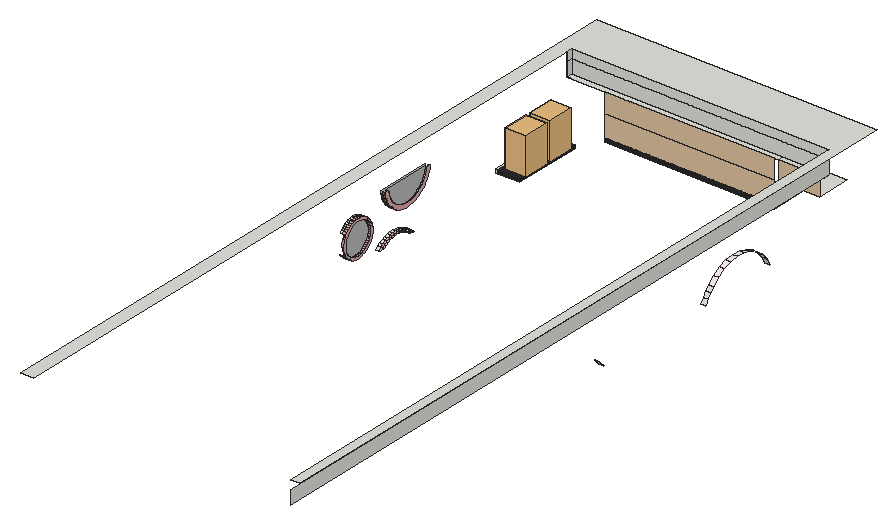
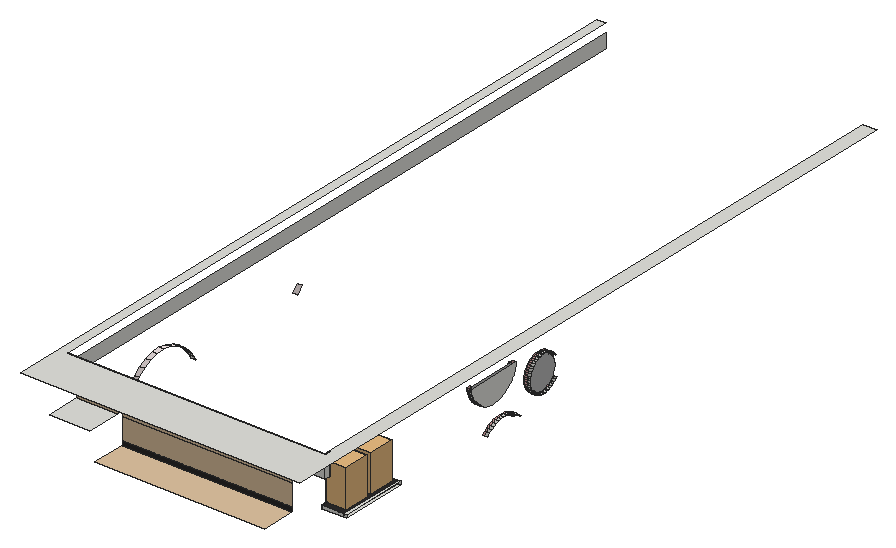
# SketchUp Ruby script. Lengths in inches.
U = 1.inch
M = Sketchup.active_model
def pt(a) = Geom::Point3d.new(a.map { |v| v * U })
def face(e, loops, mat)
  f = e.add_face(loops[0].map { |a| pt(a) })
  loops[1..].each { |l| e.add_face(l.map { |a| pt(a) }).erase! }
  f.material = f.back_material = mat if mat
  f
end
# faces: each face lists its corners as indices into pts; further lists are holes
def faces(e, pts, list, mat = nil) = list.each { |f| face(e, (f[0].is_a?(Array) ? f : [f]).map { |l| l.map { |i| pts[i] } }, mat) }
# xy, xz, yz: faces in a plane at the given z, y or x. An outline is a flat list of corners, or four numbers for a rectangle; further outlines are holes
def ring(l) = l.size == 4 ? [[l[0], l[1]], [l[2], l[1]], [l[2], l[3]], [l[0], l[3]]] : l.each_slice(2).to_a
def flat(e, list, mat, &to3) = list.each { |f| face(e, (f[0].is_a?(Array) ? f : [f]).map { |l| ring(l).map { |u, v| to3.(u, v) } }, mat) }
def xy(e, z, list, mat = nil) = flat(e, list, mat) { |x, y| [x, y, z] }
def xz(e, y, list, mat = nil) = flat(e, list, mat) { |x, z| [x, y, z] }
def yz(e, x, list, mat = nil) = flat(e, list, mat) { |y, z| [x, y, z] }
def lines(e, pts, list) = list.each { |a, b| e.add_line(pt(pts[a]), pt(pts[b])) }
# prism: a flat outline (further loops are holes) pulled along v
def prism(e, loops, v, mat = nil)
  f = face(e, loops, mat); d = Geom::Vector3d.new(v.map { |x| x * U })
  f.pushpull(f.normal.samedirection?(d) ? d.length : -d.length)
end
def box(e, o, s, mat = nil) = prism(e, [[o, [o[0] + s[0], o[1], o[2]], [o[0] + s[0], o[1] + s[1], o[2]], [o[0], o[1] + s[1], o[2]]]], [0, 0, s[2]], mat)
def at(x, y, z, deg = 0) = Geom::Transformation.translation(pt([x, y, z])) * Geom::Transformation.rotation(ORIGIN, Z_AXIS, deg.degrees)
def axes(o, x, y, z) = Geom::Transformation.new([*x, 0, *y, 0, *z, 0, *pt(o).to_a, 1])
def part(name) = M.definitions.add(name)
# library, detail: a bought-in or finely detailed component or shape, given as its bounding box
def library(name, o, s) = part(name).tap { |d| box(d.entities, o, s) }
def detail(e, o, s) = box(e.add_group.entities, o, s)
def put(e, d, t, mat = nil) = e.add_instance(d, t).tap { |i| i.material = mat if mat }
def group(e, t, mat = nil) = e.add_group.tap { |g| g.transformation = t; g.material = mat if mat }.entities
root = M.entities
M.materials.add("Generic").color = [224, 169, 169]
M.materials.add("Generic\#1").color = [44, 42, 42]
M.materials.add("Generic\#2").color = [246, 234, 234]
M.materials.add("Generic\#3").color = [224, 196, 161]
M.materials.add("[Mirror 01]").color = [185, 185, 185]
c1 = library("Untitled (9)",[-0.59,0,0],[15.67,17.07,16.5])
xy(root,88.25,[[9,393.02,10.6875,439.14]])
xy(root,88.25,[[10.6875,393.02,25.625,439.14]],"Generic\#1")
xy(root,89.18,[[34.875,453.375,150.375,476.6875]],"Generic\#3")
xy(root,90.4375,[[9,393.02,10.6875,439.14]])
xy(root,90.4375,[[10.6875,393.02,25.625,439.14]],"Generic\#1")
xy(root,107.14,[[153.2,453.375,180.77,476.9375]])
xy(root,120,[[10.6875,453.375,153.2,453.375,153.2,457.3,9,457.3,9,453.625,10.6875,453.625],[9,453.375,10.6875,453.625],[153.2,453.375,184.0625,457.3]])
xy(root,135.25,[[184.0625,0,190,0,190,490.125,0,490.125,0,0.4375,9,0.4375,9,457.3,184.0625,457.3]])
xz(root,393.02,[[9,88.25,10.6875,90.4375]])
xz(root,393.02,[[10.6875,88.25,25.625,90.4375]],"Generic\#1")
xz(root,439.14,[[9,88.25,10.6875,90.4375],[10.6875,88.25,25.625,90.4375]])
xz(root,453.375,[[34.875,89.18,149.93,92.07]],"Generic\#1")
xz(root,453.375,[[34.875,92.07,149.93,106.62],[34.875,106.62,149.93,120],[153.2,107.14,180.77,120]],"Generic\#3")
xz(root,457.3,[[9,120,184.0625,129.25],[9,129.25,184.0625,135.25]])
yz(root,9,[[314.19,103.09,315.21,103.12,316.22,103.2,317.23,103.34,318.23,103.52,319.22,103.77,320.19,104.06,321.15,104.41,322.09,104.8,323,105.25,323.89,105.74,324.75,106.28,325.59,106.87,326.39,107.5,327.15,108.17,327.88,108.875,328.57,109.625,329.22,110.41,329.82,111.23,330.38,112.07,330.9,112.95,331.37,113.85,331.79,114.78,332.15,115.73,332.47,116.7,332.74,117.68,332.95,118.67,333.16,120,295.22,120,295.4375,118.67,295.65,117.68,295.91,116.7,296.23,115.73,296.6,114.78,297.02,113.85,297.49,112.95,298,112.07,298.56,111.23,299.17,110.41,299.82,109.625,300.51,108.875,301.24,108.17,302,107.5,302.8,106.87,303.63,106.28,304.49,105.74,305.38,105.25,306.3,104.8,307.24,104.41,308.19,104.06,309.17,103.77,310.15,103.52,311.15,103.34,312.16,103.2,313.18,103.12],[453.375,120,453.625,129.25],[453.625,120,457.3,129.25],[453.375,129.25,453.625,135.25],[453.625,129.25,457.3,135.25]])
yz(root,10.6875,[[271.54,91.83,272.78,91.92,274,92.15,275.18,92.52,276.32,93.03,277.39,93.66,278.38,94.4,279.28,95.26,280.08,96.21,280.76,97.25,281.32,98.36,281.75,99.52,282.04,100.73,282.2,101.96,282.21,103.2,282.08,104.4375,281.8125,105.65,281.41,106.82,280.875,107.94,280.21,109,279.4375,109.97,278.56,110.84,277.58,111.61,276.53,112.26,275.4,112.79,274.23,113.1875,273.01,113.45,271.78,113.57,270.53,113.54,269.3,113.38,268.1,113.08,266.9375,112.64,265.83,112.07,264.8,111.38,263.85,110.58,263,109.67,262.26,108.68,261.64,107.6,261.14,106.47,260.78,105.28,260.56,104.06,260.47,102.82,260.53,101.58,260.73,100.35,261.07,99.16,261.54,98.01,262.14,96.92,262.85,95.91,263.68,94.98,264.61,94.16,265.63,93.45,266.72,92.86,267.875,92.39,269.07,92.07,270.3,91.875],[314.19,105.5625,315.08,105.59,315.96,105.66,316.84,105.77,317.71,105.9375,318.57,106.15,319.42,106.41,320.25,106.71,321.07,107.05,321.86,107.4375,322.64,107.87,323.39,108.34,324.11,108.85,324.81,109.4,325.47,109.98,326.11,110.6,326.71,111.25,327.27,111.93,327.8,112.64,328.29,113.38,328.74,114.14,329.14,114.93,329.51,115.74,329.83,116.5625,330.11,117.4,330.34,118.26,330.52,119.125,330.66,120,297.72,120,297.86,119.125,298.05,118.26,298.28,117.4,298.56,116.5625,298.88,115.74,299.24,114.93,299.65,114.14,300.1,113.38,300.59,112.64,301.12,111.93,301.68,111.25,302.28,110.6,302.91,109.98,303.58,109.4,304.28,108.85,305,108.34,305.75,107.87,306.52,107.4375,307.32,107.05,308.14,106.71,308.97,106.41,309.82,106.15,310.68,105.9375,311.55,105.77,312.43,105.66,313.31,105.59]],"[Mirror 01]")
yz(root,12.1875,[[314.19,103.09,315.21,103.12,316.22,103.2,317.23,103.34,318.23,103.52,319.22,103.77,320.19,104.06,321.15,104.41,322.09,104.8,323,105.25,323.89,105.74,324.75,106.28,325.59,106.87,326.39,107.5,327.15,108.17,327.88,108.875,328.57,109.625,329.22,110.41,329.82,111.23,330.38,112.07,330.9,112.95,331.37,113.85,331.79,114.78,332.15,115.73,332.47,116.7,332.74,117.68,332.95,118.67,333.16,120,330.66,120,330.52,119.125,330.34,118.26,330.11,117.4,329.83,116.5625,329.51,115.74,329.14,114.93,328.74,114.14,328.29,113.38,327.8,112.64,327.27,111.93,326.71,111.25,326.11,110.6,325.47,109.98,324.81,109.4,324.11,108.85,323.39,108.34,322.64,107.87,321.86,107.4375,321.07,107.05,320.25,106.71,319.42,106.41,318.57,106.15,317.71,105.9375,316.84,105.77,315.96,105.66,315.08,105.59,314.19,105.5625,313.31,105.59,312.43,105.66,311.55,105.77,310.68,105.9375,309.82,106.15,308.97,106.41,308.14,106.71,307.32,107.05,306.52,107.4375,305.75,107.87,305,108.34,304.28,108.85,303.58,109.4,302.91,109.98,302.28,110.6,301.68,111.25,301.12,111.93,300.59,112.64,300.1,113.38,299.65,114.14,299.24,114.93,298.88,115.74,298.56,116.5625,298.28,117.4,298.05,118.26,297.86,119.125,297.72,120,295.22,120,295.4375,118.67,295.65,117.68,295.91,116.7,296.23,115.73,296.6,114.78,297.02,113.85,297.49,112.95,298,112.07,298.56,111.23,299.17,110.41,299.82,109.625,300.51,108.875,301.24,108.17,302,107.5,302.8,106.87,303.63,106.28,304.49,105.74,305.38,105.25,306.3,104.8,307.24,104.41,308.19,104.06,309.17,103.77,310.15,103.52,311.15,103.34,312.16,103.2,313.18,103.12]],"Generic")
yz(root,12.9375,[[[271.5625,90.52,272.95,90.625,274.32,90.89,275.64,91.3,276.91,91.86,278.11,92.57,279.22,93.41,280.23,94.37,281.125,95.43,281.89,96.59,282.52,97.84,283,99.14,283.33,100.49,283.5,101.87,283.52,103.26,283.37,104.65,283.07,106,282.62,107.32,282.02,108.57,281.28,109.75,280.41,110.84,279.42,111.82,278.33,112.68,277.15,113.41,275.89,114,274.57,114.45,273.21,114.74,271.83,114.87,270.4375,114.85,269.06,114.66,267.71,114.32,266.41,113.83,265.17,113.2,264.01,112.43,262.95,111.53,262,110.51,261.17,109.4,260.47,108.19,259.92,106.92,259.51,105.59,259.26,104.22,259.17,102.83,259.23,101.44,259.45,100.07,259.83,98.73,260.36,97.44,261.03,96.23,261.83,95.09,262.76,94.06,263.8,93.13,264.94,92.34,266.17,91.67,267.46,91.16,268.8,90.79,270.17,90.58],[271.54,91.83,270.3,91.875,269.07,92.07,267.875,92.39,266.72,92.86,265.63,93.45,264.61,94.16,263.68,94.98,262.85,95.91,262.14,96.92,261.54,98.01,261.07,99.16,260.73,100.35,260.53,101.58,260.47,102.82,260.56,104.06,260.78,105.28,261.14,106.47,261.64,107.6,262.26,108.68,263,109.67,263.85,110.58,264.8,111.38,265.83,112.07,266.9375,112.64,268.1,113.08,269.3,113.38,270.53,113.54,271.78,113.57,273.01,113.45,274.23,113.1875,275.4,112.79,276.53,112.26,277.58,111.61,278.56,110.84,279.4375,109.97,280.21,109,280.875,107.94,281.41,106.82,281.8125,105.65,282.08,104.4375,282.21,103.2,282.2,101.96,282.04,100.73,281.75,99.52,281.32,98.36,280.76,97.25,280.08,96.21,279.28,95.26,278.38,94.4,277.39,93.66,276.32,93.03,275.18,92.52,274,92.15,272.78,91.92]]],"Generic")
yz(root,25.625,[[393.02,88.25,439.14,90.4375]],"Generic\#1")
yz(root,184.0625,[[0,120,457.3,129.25]])
p = [[10.6875,319.64,85.27],[10.6875,318.02,86.82],[9,318.02,86.82],[9,319.64,85.27],[12,318.02,86.82],[12,319.64,85.27],
  [10.6875,315.38,86.91],[10.6875,317.03,85.66],[12,317.03,85.66],[12,315.38,86.91],[10.6875,293.15,87.33],[10.6875,291.47,85.85],
  [9,291.47,85.85],[9,293.15,87.33],[12,291.47,85.85],[12,293.15,87.33],[10.6875,294.09,86.13],[10.6875,295.79,87.3125],
  [12,295.79,87.3125],[12,294.09,86.13],[184.0625,354.54,89.43],[184.0625,352.42,86.46],[180.9375,352.42,86.46],[180.9375,354.54,89.43],
  [10.6875,316.23,88.17],[9,316.23,88.17],[12,316.23,88.17],[10.6875,313.6,87.96],[12,313.6,87.96],[184.0625,406.96,87.1875],
  [184.0625,404.1875,92.23],[180.9375,404.1875,92.23],[180.9375,406.96,87.1875],[10.6875,294.99,88.61],[9,294.99,88.61],[12,294.99,88.61],
  [10.6875,297.61,88.29],[12,297.61,88.29],[184.0625,265.88,87.89],[184.0625,262.21,91.98],[180.9375,262.21,91.98],[180.9375,265.88,87.89],
  [10.6875,311.71,88.81],[12,311.71,88.81],[10.6875,314.3,89.31],[9,314.3,89.31],[12,314.3,89.31],[10.6875,299.53,89.06],
  [12,299.53,89.06],[10.6875,296.97,89.67],[9,296.97,89.67],[12,296.97,89.67],[10.6875,309.74,89.43],[12,309.74,89.43],
  [10.6875,301.53,89.6],[12,301.53,89.6],[10.6875,312.25,90.23],[9,312.25,90.23],[12,312.25,90.23],[10.6875,307.71,89.83],
  [12,307.71,89.83],[184.0625,356.78,92.31],[180.9375,356.78,92.31],[10.6875,303.58,89.91],[12,303.58,89.91],[10.6875,299.05,90.5],
  [9,299.05,90.5],[12,299.05,90.5],[10.6875,305.64,89.99],[12,305.64,89.99],[10.6875,310.11,90.91],[9,310.11,90.91],
  [12,310.11,90.91],[10.6875,270.17,90.58],[10.6875,271.5625,90.52],[9,271.5625,90.52],[9,270.17,90.58],[12.9375,271.5625,90.52],
  [12.9375,270.17,90.58],[10.6875,272.95,90.625],[9,272.95,90.625],[12.9375,272.95,90.625],[10.6875,301.22,91.09],[9,301.22,91.09],
  [12,301.22,91.09],[10.6875,268.8,90.79],[9,268.8,90.79],[12.9375,268.8,90.79],[10.6875,274.32,90.89],[9,274.32,90.89],
  [12.9375,274.32,90.89],[10.6875,267.46,91.16],[9,267.46,91.16],[12.9375,267.46,91.16],[10.6875,275.64,91.3],[9,275.64,91.3],
  [12.9375,275.64,91.3],[10.6875,307.91,91.33],[9,307.91,91.33],[12,307.91,91.33],[10.6875,303.43,91.43],[9,303.43,91.43],
  [12,303.43,91.43],[10.6875,266.17,91.67],[9,266.17,91.67],[12.9375,266.17,91.67],[10.6875,276.91,91.86],[9,276.91,91.86],
  [12.9375,276.91,91.86],[10.6875,305.68,91.51],[9,305.68,91.51],[12,305.68,91.51],[10.6875,264.94,92.34],[9,264.94,92.34],
  [12.9375,264.94,92.34],[10.6875,271.54,91.83],[10.6875,270.3,91.875],[12.9375,270.3,91.875],[12.9375,271.54,91.83],[10.6875,272.78,91.92],
  [12.9375,272.78,91.92],[10.6875,269.07,92.07],[12.9375,269.07,92.07],[10.6875,274,92.15],[12.9375,274,92.15],[10.6875,278.11,92.57],
  [9,278.11,92.57],[12.9375,278.11,92.57],[10.6875,267.875,92.39],[12.9375,267.875,92.39],[10.6875,275.18,92.52],[12.9375,275.18,92.52],
  [184.0625,400.46,96.625],[180.9375,400.46,96.625],[10.6875,263.8,93.13],[9,263.8,93.13],[12.9375,263.8,93.13],[184.0625,359.15,95.08],
  [180.9375,359.15,95.08],[10.6875,266.72,92.86],[12.9375,266.72,92.86],[10.6875,276.32,93.03],[12.9375,276.32,93.03],[10.6875,279.22,93.41],
  [9,279.22,93.41],[12.9375,279.22,93.41],[10.6875,265.63,93.45],[12.9375,265.63,93.45],[10.6875,277.39,93.66],[12.9375,277.39,93.66],
  [10.6875,262.76,94.06],[9,262.76,94.06],[12.9375,262.76,94.06],[10.6875,264.61,94.16],[12.9375,264.61,94.16],[10.6875,280.23,94.37],
  [9,280.23,94.37],[12.9375,280.23,94.37],[10.6875,278.38,94.4],[12.9375,278.38,94.4],[10.6875,261.83,95.09],[9,261.83,95.09],
  [12.9375,261.83,95.09],[10.6875,263.68,94.98],[12.9375,263.68,94.98],[10.6875,279.28,95.26],[12.9375,279.28,95.26],[10.6875,281.125,95.43],
  [9,281.125,95.43],[12.9375,281.125,95.43],[10.6875,262.85,95.91],[12.9375,262.85,95.91],[10.6875,261.03,96.23],[9,261.03,96.23],
  [12.9375,261.03,96.23],[184.0625,363.4,98.97],[180.9375,363.4,98.97],[10.6875,280.08,96.21],[12.9375,280.08,96.21],[10.6875,281.89,96.59],
  [9,281.89,96.59],[12.9375,281.89,96.59],[10.6875,262.14,96.92],[12.9375,262.14,96.92],[10.6875,280.76,97.25],[12.9375,280.76,97.25],
  [10.6875,282.52,97.84],[9,282.52,97.84],[12.9375,282.52,97.84],[184.0625,395.93,100.18],[180.9375,395.93,100.18],[10.6875,261.54,98.01],
  [12.9375,261.54,98.01],[10.6875,281.32,98.36],[12.9375,281.32,98.36],[10.6875,283,99.14],[9,283,99.14],[12.9375,283,99.14],
  [10.6875,261.07,99.16],[12.9375,261.07,99.16],[10.6875,281.75,99.52],[12.9375,281.75,99.52],[184.0625,368.34,101.93],[180.9375,368.34,101.93],
  [10.6875,283.33,100.49],[9,283.33,100.49],[12.9375,283.33,100.49],[10.6875,282.04,100.73],[12.9375,282.04,100.73],[184.0625,390.79,102.77],
  [180.9375,390.79,102.77],[10.6875,283.5,101.87],[9,283.5,101.87],[12.9375,283.5,101.87],[10.6875,282.2,101.96],[12.9375,282.2,101.96],
  [10.6875,283.52,103.26],[9,283.52,103.26],[12.9375,283.52,103.26],[184.0625,373.77,103.84],[180.9375,373.77,103.84],[10.6875,282.21,103.2],
  [12.9375,282.21,103.2],[184.0625,385.23,104.27],[180.9375,385.23,104.27],[10.6875,312.16,103.2],[10.6875,313.18,103.12],[9,313.18,103.12],
  [9,312.16,103.2],[12.1875,313.18,103.12],[12.1875,312.16,103.2],[10.6875,314.19,103.09],[9,314.19,103.09],[12.1875,314.19,103.09],
  [10.6875,315.21,103.12],[9,315.21,103.12],[12.1875,315.21,103.12],[10.6875,316.22,103.2],[9,316.22,103.2],[12.1875,316.22,103.2],
  [10.6875,282.08,104.4375],[12.9375,282.08,104.4375],[10.6875,311.15,103.34],[9,311.15,103.34],[12.1875,311.15,103.34],[10.6875,317.23,103.34],
  [9,317.23,103.34],[12.1875,317.23,103.34],[10.6875,283.37,104.65],[9,283.37,104.65],[12.9375,283.37,104.65],[10.6875,310.15,103.52],
  [9,310.15,103.52],[12.1875,310.15,103.52],[10.6875,318.23,103.52],[9,318.23,103.52],[12.1875,318.23,103.52],[10.6875,309.17,103.77],
  [9,309.17,103.77],[12.1875,309.17,103.77],[10.6875,319.22,103.77],[9,319.22,103.77],[12.1875,319.22,103.77],[10.6875,308.19,104.06],
  [9,308.19,104.06],[12.1875,308.19,104.06],[10.6875,320.19,104.06],[9,320.19,104.06],[12.1875,320.19,104.06],[184.0625,379.48,104.64],
  [180.9375,379.48,104.64],[10.6875,307.24,104.41],[9,307.24,104.41],[12.1875,307.24,104.41],[10.6875,321.15,104.41],[9,321.15,104.41],
  [12.1875,321.15,104.41],[10.6875,281.8125,105.65],[12.9375,281.8125,105.65],[10.6875,306.3,104.8],[9,306.3,104.8],[12.1875,306.3,104.8],
  [10.6875,322.09,104.8],[9,322.09,104.8],[12.1875,322.09,104.8],[10.6875,283.07,106],[9,283.07,106],[12.9375,283.07,106],
  [10.6875,305.38,105.25],[9,305.38,105.25],[12.1875,305.38,105.25],[10.6875,323,105.25],[9,323,105.25],[12.1875,323,105.25],
  [10.6875,304.49,105.74],[9,304.49,105.74],[12.1875,304.49,105.74],[10.6875,323.89,105.74],[9,323.89,105.74],[12.1875,323.89,105.74],
  [10.6875,281.41,106.82],[12.9375,281.41,106.82],[10.6875,313.31,105.59],[10.6875,312.43,105.66],[12.1875,312.43,105.66],[12.1875,313.31,105.59],
  [10.6875,314.19,105.5625],[12.1875,314.19,105.5625],[10.6875,315.08,105.59],[12.1875,315.08,105.59],[10.6875,315.96,105.66],[12.1875,315.96,105.66],
  [10.6875,303.63,106.28],[9,303.63,106.28],[12.1875,303.63,106.28],[10.6875,311.55,105.77],[12.1875,311.55,105.77],[10.6875,316.84,105.77],
  [12.1875,316.84,105.77],[10.6875,324.75,106.28],[9,324.75,106.28],[12.1875,324.75,106.28],[10.6875,310.68,105.9375],[12.1875,310.68,105.9375],
  [10.6875,317.71,105.9375],[12.1875,317.71,105.9375],[10.6875,309.82,106.15],[12.1875,309.82,106.15],[10.6875,318.57,106.15],[12.1875,318.57,106.15],
  [10.6875,282.62,107.32],[9,282.62,107.32],[12.9375,282.62,107.32],[10.6875,308.97,106.41],[12.1875,308.97,106.41],[10.6875,319.42,106.41],
  [12.1875,319.42,106.41],[10.6875,302.8,106.87],[9,302.8,106.87],[12.1875,302.8,106.87],[10.6875,325.59,106.87],[9,325.59,106.87],
  [12.1875,325.59,106.87],[10.6875,308.14,106.71],[12.1875,308.14,106.71],[10.6875,320.25,106.71],[12.1875,320.25,106.71],[10.6875,261.14,106.47],
  [10.6875,261.64,107.6],[12.9375,261.64,107.6],[12.9375,261.14,106.47],[10.6875,307.32,107.05],[12.1875,307.32,107.05],[10.6875,321.07,107.05],
  [12.1875,321.07,107.05],[10.6875,280.875,107.94],[12.9375,280.875,107.94],[10.6875,302,107.5],[9,302,107.5],[12.1875,302,107.5],
  [10.6875,326.39,107.5],[9,326.39,107.5],[12.1875,326.39,107.5],[10.6875,306.52,107.4375],[12.1875,306.52,107.4375],[10.6875,321.86,107.4375],
  [12.1875,321.86,107.4375],[10.6875,282.02,108.57],[9,282.02,108.57],[12.9375,282.02,108.57],[10.6875,305.75,107.87],[12.1875,305.75,107.87],
  [10.6875,322.64,107.87],[12.1875,322.64,107.87],[10.6875,301.24,108.17],[9,301.24,108.17],[12.1875,301.24,108.17],[10.6875,327.15,108.17],
  [9,327.15,108.17],[12.1875,327.15,108.17],[10.6875,262.26,108.68],[12.9375,262.26,108.68],[10.6875,280.21,109],[12.9375,280.21,109],
  [10.6875,305,108.34],[12.1875,305,108.34],[10.6875,323.39,108.34],[12.1875,323.39,108.34],[10.6875,300.51,108.875],[9,300.51,108.875],
  [12.1875,300.51,108.875],[10.6875,327.88,108.875],[9,327.88,108.875],[12.1875,327.88,108.875],[10.6875,304.28,108.85],[12.1875,304.28,108.85],
  [10.6875,324.11,108.85],[12.1875,324.11,108.85],[10.6875,281.28,109.75],[9,281.28,109.75],[12.9375,281.28,109.75],[10.6875,263,109.67],
  [12.9375,263,109.67],[10.6875,303.58,109.4],[12.1875,303.58,109.4],[10.6875,324.81,109.4],[12.1875,324.81,109.4],[10.6875,299.82,109.625],
  [9,299.82,109.625],[12.1875,299.82,109.625],[10.6875,328.57,109.625],[9,328.57,109.625],[12.1875,328.57,109.625],[10.6875,279.4375,109.97],
  [12.9375,279.4375,109.97],[10.6875,262,110.51],[10.6875,261.17,109.4],[9,261.17,109.4],[9,262,110.51],[12.9375,261.17,109.4],
  [12.9375,262,110.51],[10.6875,302.91,109.98],[12.1875,302.91,109.98],[10.6875,325.47,109.98],[12.1875,325.47,109.98],[10.6875,299.17,110.41],
  [9,299.17,110.41],[12.1875,299.17,110.41],[10.6875,329.22,110.41],[9,329.22,110.41],[12.1875,329.22,110.41],[10.6875,263.85,110.58],
  [12.9375,263.85,110.58],[10.6875,280.41,110.84],[9,280.41,110.84],[12.9375,280.41,110.84],[10.6875,278.56,110.84],[12.9375,278.56,110.84],
  [10.6875,302.28,110.6],[12.1875,302.28,110.6],[10.6875,326.11,110.6],[12.1875,326.11,110.6],[10.6875,298.56,111.23],[9,298.56,111.23],
  [12.1875,298.56,111.23],[10.6875,329.82,111.23],[9,329.82,111.23],[12.1875,329.82,111.23],[10.6875,262.95,111.53],[9,262.95,111.53],
  [12.9375,262.95,111.53],[10.6875,264.8,111.38],[12.9375,264.8,111.38],[10.6875,301.68,111.25],[12.1875,301.68,111.25],[10.6875,326.71,111.25],
  [12.1875,326.71,111.25],[10.6875,277.58,111.61],[12.9375,277.58,111.61],[10.6875,279.42,111.82],[9,279.42,111.82],[12.9375,279.42,111.82],
  [10.6875,298,112.07],[9,298,112.07],[12.1875,298,112.07],[10.6875,301.12,111.93],[12.1875,301.12,111.93],[10.6875,327.27,111.93],
  [12.1875,327.27,111.93],[10.6875,330.38,112.07],[9,330.38,112.07],[12.1875,330.38,112.07],[10.6875,265.83,112.07],[12.9375,265.83,112.07],
  [10.6875,264.01,112.43],[9,264.01,112.43],[12.9375,264.01,112.43],[10.6875,276.53,112.26],[12.9375,276.53,112.26],[10.6875,278.33,112.68],
  [9,278.33,112.68],[12.9375,278.33,112.68],[10.6875,300.59,112.64],[12.1875,300.59,112.64],[10.6875,327.8,112.64],[12.1875,327.8,112.64],
  [10.6875,266.9375,112.64],[12.9375,266.9375,112.64],[10.6875,297.49,112.95],[9,297.49,112.95],[12.1875,297.49,112.95],[10.6875,330.9,112.95],
  [9,330.9,112.95],[12.1875,330.9,112.95],[10.6875,275.4,112.79],[12.9375,275.4,112.79],[10.6875,265.17,113.2],[9,265.17,113.2],
  [12.9375,265.17,113.2],[10.6875,268.1,113.08],[12.9375,268.1,113.08],[10.6875,300.1,113.38],[12.1875,300.1,113.38],[10.6875,328.29,113.38],
  [12.1875,328.29,113.38],[10.6875,277.15,113.41],[9,277.15,113.41],[12.9375,277.15,113.41],[10.6875,274.23,113.1875],[12.9375,274.23,113.1875],
  [10.6875,297.02,113.85],[9,297.02,113.85],[12.1875,297.02,113.85],[10.6875,331.37,113.85],[9,331.37,113.85],[12.1875,331.37,113.85],
  [10.6875,269.3,113.38],[12.9375,269.3,113.38],[10.6875,266.41,113.83],[9,266.41,113.83],[12.9375,266.41,113.83],[10.6875,273.01,113.45],
  [12.9375,273.01,113.45],[10.6875,270.53,113.54],[12.9375,270.53,113.54],[10.6875,271.78,113.57],[12.9375,271.78,113.57],[10.6875,275.89,114],
  [9,275.89,114],[12.9375,275.89,114],[10.6875,299.65,114.14],[12.1875,299.65,114.14],[10.6875,328.74,114.14],[12.1875,328.74,114.14],
  [10.6875,267.71,114.32],[9,267.71,114.32],[12.9375,267.71,114.32],[10.6875,296.6,114.78],[9,296.6,114.78],[12.1875,296.6,114.78],
  [10.6875,331.79,114.78],[9,331.79,114.78],[12.1875,331.79,114.78],[10.6875,274.57,114.45],[9,274.57,114.45],[12.9375,274.57,114.45],
  [10.6875,299.24,114.93],[12.1875,299.24,114.93],[10.6875,329.14,114.93],[12.1875,329.14,114.93],[10.6875,269.06,114.66],[9,269.06,114.66],
  [12.9375,269.06,114.66],[10.6875,273.21,114.74],[9,273.21,114.74],[12.9375,273.21,114.74],[10.6875,270.4375,114.85],[9,270.4375,114.85],
  [12.9375,270.4375,114.85],[10.6875,271.83,114.87],[9,271.83,114.87],[12.9375,271.83,114.87],[10.6875,296.23,115.73],[9,296.23,115.73],
  [12.1875,296.23,115.73],[10.6875,332.15,115.73],[9,332.15,115.73],[12.1875,332.15,115.73],[10.6875,298.88,115.74],[12.1875,298.88,115.74],
  [10.6875,329.51,115.74],[12.1875,329.51,115.74],[10.6875,295.91,116.7],[9,295.91,116.7],[12.1875,295.91,116.7],[10.6875,298.56,116.5625],
  [12.1875,298.56,116.5625],[10.6875,329.83,116.5625],[12.1875,329.83,116.5625],[10.6875,332.47,116.7],[9,332.47,116.7],[12.1875,332.47,116.7],
  [10.6875,298.28,117.4],[12.1875,298.28,117.4],[10.6875,330.11,117.4],[12.1875,330.11,117.4],[10.6875,295.65,117.68],[9,295.65,117.68],
  [12.1875,295.65,117.68],[10.6875,332.74,117.68],[9,332.74,117.68],[12.1875,332.74,117.68],[10.6875,298.05,118.26],[12.1875,298.05,118.26],
  [10.6875,330.34,118.26],[12.1875,330.34,118.26],[10.6875,295.4375,118.67],[9,295.4375,118.67],[12.1875,295.4375,118.67],[10.6875,332.95,118.67],
  [9,332.95,118.67],[12.1875,332.95,118.67],[10.6875,297.86,119.125],[12.1875,297.86,119.125],[10.6875,330.52,119.125],[12.1875,330.52,119.125],
  [10.6875,295.22,120],[12.1875,295.22,120],[10.6875,333.16,120],[12.1875,333.16,120],[10.6875,297.72,120],[12.1875,297.72,120],
  [10.6875,330.66,120],[12.1875,330.66,120]]
faces(root,p,[[0,1,2,3],[10,11,12,13],[20,21,22,23],[1,24,25,2],[33,10,13,34],[24,44,45,25],[49,33,34,50],[44,56,57,45],
  [61,20,23,62],[65,49,50,66],[56,70,71,57],[73,74,75,76],[74,79,80,75],[82,65,66,83],[85,73,76,86],[79,88,89,80],
  [91,85,86,92],[88,94,95,89],[70,97,98,71],[100,82,83,101],[103,91,92,104],[94,106,107,95],[97,109,110,98],[109,100,101,110],
  [112,103,104,113],[106,125,126,107],[134,112,113,135],[137,61,62,138],[125,143,144,126],[150,134,135,151],[143,155,156,144],[160,150,151,161],
  [155,167,168,156],[172,160,161,173],[167,179,180,168],[179,186,187,180],[186,195,196,187],[195,204,205,196],[204,211,212,205],[211,216,217,212],
  [225,226,227,228],[226,231,232,227],[231,234,235,232],[234,237,238,235],[242,225,228,243],[237,245,246,238],[216,248,249,217],[251,242,243,252],
  [245,254,255,246],[257,251,252,258],[254,260,261,255],[263,257,258,264],[260,266,267,261],[271,263,264,272],[266,274,275,267],[279,271,272,280],
  [274,282,283,275],[248,285,286,249],[288,279,280,289],[282,291,292,283],[294,288,289,295],[291,297,298,292],[312,294,295,313],[297,319,320,298],
  [285,330,331,286],[337,312,313,338],[319,340,341,320],[357,337,338,358],[340,360,361,341],[330,367,368,331],[374,357,358,375],[360,377,378,361],
  [388,374,375,389],[377,391,392,378],[367,398,399,368],[407,388,389,408],[391,410,411,392],[415,416,417,418],[425,407,408,426],[410,428,429,411],
  [398,433,434,399],[442,425,426,443],[428,445,446,429],[448,415,418,449],[433,459,460,434],[462,442,443,463],[445,469,470,446],[474,448,449,475],
  [459,479,480,460],[488,462,463,489],[469,491,492,470],[496,474,475,497],[479,505,506,480],[510,488,489,511],[491,513,514,492],[518,496,497,519],
  [505,527,528,506],[534,518,519,535],[537,510,511,538],[513,540,541,514],[527,543,544,528],[550,534,535,551],[543,553,554,544],[556,550,551,557],
  [553,559,560,554],[559,556,557,560],[562,537,538,563],[540,565,566,541],[572,562,563,573],[565,579,580,566],[586,572,573,587],[579,589,590,580],
  [596,586,587,597],[589,599,600,590]])
faces(root,p,[[0,1,4,5],[6,7,8,9],[10,11,14,15],[16,17,18,19],[1,24,26,4],[27,6,9,28],[33,10,15,35],[17,36,37,18],
  [42,27,28,43],[24,44,46,26],[36,47,48,37],[49,33,35,51],[52,42,43,53],[47,54,55,48],[44,56,58,46],[59,52,53,60],
  [54,63,64,55],[65,49,51,67],[68,59,60,69],[63,68,69,64],[56,70,72,58],[73,74,77,78],[74,79,81,77],[82,65,67,84],
  [85,73,78,87],[79,88,90,81],[91,85,87,93],[88,94,96,90],[70,97,99,72],[100,82,84,102],[103,91,93,105],[94,106,108,96],
  [97,109,111,99],[109,100,102,111],[112,103,105,114],[115,116,117,118],[119,115,118,120],[116,121,122,117],[123,119,120,124],[106,125,127,108],
  [121,128,129,122],[130,123,124,131],[134,112,114,136],[128,139,140,129],[141,130,131,142],[125,143,145,127],[139,146,147,140],[148,141,142,149],
  [150,134,136,152],[146,153,154,147],[143,155,157,145],[158,148,149,159],[160,150,152,162],[153,163,164,154],[165,158,159,166],[155,167,169,157],
  [163,170,171,164],[172,160,162,174],[177,165,166,178],[167,179,181,169],[170,182,183,171],[184,177,178,185],[179,186,188,181],[182,191,192,183],
  [193,184,185,194],[186,195,197,188],[191,198,199,192],[200,193,194,201],[195,204,206,197],[207,200,201,208],[204,211,213,206],[214,207,208,215],
  [211,216,218,213],[221,214,215,222],[225,226,229,230],[226,231,233,229],[231,234,236,233],[234,237,239,236],[240,221,222,241],[242,225,230,244],
  [237,245,247,239],[216,248,250,218],[251,242,244,253],[245,254,256,247],[257,251,253,259],[254,260,262,256],[263,257,259,265],[260,266,268,262],
  [271,263,265,273],[266,274,276,268],[277,240,241,278],[279,271,273,281],[274,282,284,276],[248,285,287,250],[288,279,281,290],[282,291,293,284],
  [294,288,290,296],[291,297,299,293],[300,277,278,301],[302,303,304,305],[306,302,305,307],[308,306,307,309],[310,308,309,311],[312,294,296,314],
  [303,315,316,304],[317,310,311,318],[297,319,321,299],[315,322,323,316],[324,317,318,325],[322,326,327,323],[328,324,325,329],[285,330,332,287],
  [326,333,334,327],[335,328,329,336],[337,312,314,339],[319,340,342,321],[333,343,344,334],[345,335,336,346],[347,348,349,350],[343,351,352,344],
  [353,345,346,354],[355,300,301,356],[357,337,339,359],[340,360,362,342],[351,363,364,352],[365,353,354,366],[330,367,369,332],[363,370,371,364],
  [372,365,366,373],[374,357,359,376],[360,377,379,362],[348,380,381,349],[382,355,356,383],[370,384,385,371],[386,372,373,387],[388,374,376,390],
  [377,391,393,379],[384,394,395,385],[396,386,387,397],[367,398,400,369],[380,401,402,381],[394,403,404,395],[405,396,397,406],[407,388,390,409],
  [391,410,412,393],[413,382,383,414],[415,416,419,420],[403,421,422,404],[423,405,406,424],[425,407,409,427],[410,428,430,412],[401,431,432,402],
  [398,433,435,400],[436,413,414,437],[421,438,439,422],[440,423,424,441],[442,425,427,444],[428,445,447,430],[448,415,420,450],[431,451,452,432],
  [438,453,454,439],[455,440,441,456],[457,436,437,458],[433,459,461,435],[462,442,444,464],[453,465,466,454],[467,455,456,468],[445,469,471,447],
  [451,472,473,452],[474,448,450,476],[477,457,458,478],[459,479,481,461],[465,482,483,466],[484,467,468,485],[472,486,487,473],[488,462,464,490],
  [469,491,493,471],[494,477,478,495],[496,474,476,498],[486,499,500,487],[482,501,502,483],[503,484,485,504],[479,505,507,481],[508,494,495,509],
  [510,488,490,512],[491,513,515,493],[499,516,517,500],[518,496,498,520],[521,508,509,522],[516,523,524,517],[525,521,522,526],[505,527,529,507],
  [501,530,531,502],[532,503,504,533],[523,525,526,524],[534,518,520,536],[537,510,512,539],[513,540,542,515],[527,543,545,529],[530,546,547,531],
  [548,532,533,549],[550,534,536,552],[543,553,555,545],[556,550,552,558],[553,559,561,555],[559,556,558,561],[562,537,539,564],[540,565,567,542],
  [546,568,569,547],[570,548,549,571],[572,562,564,574],[568,575,576,569],[577,570,571,578],[565,579,581,567],[575,582,583,576],[584,577,578,585],
  [586,572,574,588],[579,589,591,581],[582,592,593,583],[594,584,585,595],[596,586,588,598],[589,599,601,591],[592,602,603,593],[604,594,595,605],
  [606,596,598,607],[599,608,609,601],[602,610,611,603],[612,604,605,613]],"Generic")
faces(root,p,[[29,30,31,32],[38,39,40,41],[30,132,133,31],[175,137,138,176],[132,189,190,133],[202,175,176,203],[189,209,210,190],[219,202,203,220],
  [209,223,224,210],[269,219,220,270],[223,269,270,224]],"Generic\#2")
put(root,c1,axes([26.48,413.875,90.4375],[-0.88888,0,0],[0,-1.0607,0],[0,0,1.51998]),"Generic\#1")
put(root,c1,axes([26.16,435.0625,90.4375],[-0.88888,0,0],[0,-1.0607,0],[0,0,1.51998]))
